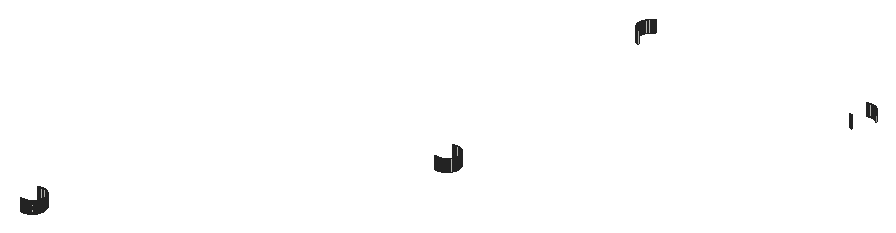
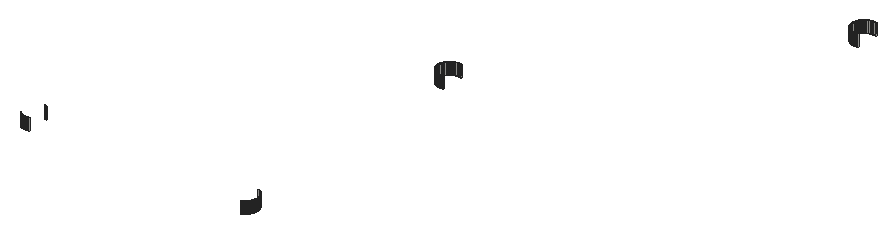
# SketchUp Ruby script. Lengths in inches.
U = 1.inch
M = Sketchup.active_model
def pt(a) = Geom::Point3d.new(a.map { |v| v * U })
def face(e, loops, mat)
  f = e.add_face(loops[0].map { |a| pt(a) })
  loops[1..].each { |l| e.add_face(l.map { |a| pt(a) }).erase! }
  f.material = f.back_material = mat if mat
  f
end
# faces: each face lists its corners as indices into pts; further lists are holes
def faces(e, pts, list, mat = nil) = list.each { |f| face(e, (f[0].is_a?(Array) ? f : [f]).map { |l| l.map { |i| pts[i] } }, mat) }
# xy, xz, yz: faces in a plane at the given z, y or x. An outline is a flat list of corners, or four numbers for a rectangle; further outlines are holes
def ring(l) = l.size == 4 ? [[l[0], l[1]], [l[2], l[1]], [l[2], l[3]], [l[0], l[3]]] : l.each_slice(2).to_a
def flat(e, list, mat, &to3) = list.each { |f| face(e, (f[0].is_a?(Array) ? f : [f]).map { |l| ring(l).map { |u, v| to3.(u, v) } }, mat) }
def xy(e, z, list, mat = nil) = flat(e, list, mat) { |x, y| [x, y, z] }
def xz(e, y, list, mat = nil) = flat(e, list, mat) { |x, z| [x, y, z] }
def yz(e, x, list, mat = nil) = flat(e, list, mat) { |y, z| [x, y, z] }
def lines(e, pts, list) = list.each { |a, b| e.add_line(pt(pts[a]), pt(pts[b])) }
# prism: a flat outline (further loops are holes) pulled along v
def prism(e, loops, v, mat = nil)
  f = face(e, loops, mat); d = Geom::Vector3d.new(v.map { |x| x * U })
  f.pushpull(f.normal.samedirection?(d) ? d.length : -d.length)
end
def box(e, o, s, mat = nil) = prism(e, [[o, [o[0] + s[0], o[1], o[2]], [o[0] + s[0], o[1] + s[1], o[2]], [o[0], o[1] + s[1], o[2]]]], [0, 0, s[2]], mat)
def at(x, y, z, deg = 0) = Geom::Transformation.translation(pt([x, y, z])) * Geom::Transformation.rotation(ORIGIN, Z_AXIS, deg.degrees)
def axes(o, x, y, z) = Geom::Transformation.new([*x, 0, *y, 0, *z, 0, *pt(o).to_a, 1])
def part(name) = M.definitions.add(name)
# library, detail: a bought-in or finely detailed component or shape, given as its bounding box
def library(name, o, s) = part(name).tap { |d| box(d.entities, o, s) }
def detail(e, o, s) = box(e.add_group.entities, o, s)
def put(e, d, t, mat = nil) = e.add_instance(d, t).tap { |i| i.material = mat if mat }
def group(e, t, mat = nil) = e.add_group.tap { |g| g.transformation = t; g.material = mat if mat }.entities
root = M.entities
xz(root,185,[[159.48,231,159.55,234],[159.55,231,159.63,234],[159.63,231,159.71,234]])
xz(root,185.01,[[159.32,231,159.4,234],[159.79,231,159.87,234]])
xz(root,190.99,[[159.33,231,159.41,234],[159.8,231,159.88,234]])
xz(root,191,[[159.49,231,159.57,234],[159.57,231,159.65,234],[159.65,231,159.72,234]])
xz(root,251,[[214.28,231,214.35,234],[214.35,231,214.43,234],[214.43,231,214.51,234]])
xz(root,251.01,[[214.12,231,214.2,234],[214.59,231,214.67,234]])
xz(root,256.99,[[214.13,231,214.21,234],[214.6,231,214.68,234]])
xz(root,257,[[214.29,231,214.37,234],[214.37,231,214.45,234],[214.45,231,214.52,234]])
xz(root,317,[[269.08,231,269.15,234]])
xz(root,317.01,[[268.92,231,269,234]])
xz(root,322.99,[[268.93,231,269.01,234],[269.4,231,269.48,234]])
xz(root,323,[[269.09,231,269.17,234],[269.17,231,269.25,234],[269.25,231,269.32,234]])
yz(root,162.59,[[187.72,231,187.8,234],[188.19,231,188.27,234]])
yz(root,162.6,[[187.875,231,187.95,234],[187.95,231,188.03,234],[188.03,231,188.11,234]])
yz(root,211.4,[[319.89,231,319.97,234],[319.97,231,320.05,234],[320.05,231,320.125,234]])
yz(root,211.41,[[319.73,231,319.81,234],[320.2,231,320.28,234]])
yz(root,217.39,[[253.72,231,253.8,234],[254.19,231,254.27,234]])
yz(root,217.4,[[253.875,231,253.95,234],[253.95,231,254.03,234],[254.03,231,254.11,234]])
p = [[159.09,185.04,231],[159.01,185.06,231],[159.01,185.06,234],[159.09,185.04,234],[159.16,185.03,231],[159.16,185.03,234],
  [159.32,185.01,231],[159.24,185.02,231],[159.24,185.02,234],[159.32,185.01,234],[159.48,185,231],[159.4,185.01,231],
  [159.4,185.01,234],[159.48,185,234],[159.79,185.01,231],[159.71,185,231],[159.71,185,234],[159.79,185.01,234],
  [160.02,185.03,231],[159.95,185.02,231],[159.95,185.02,234],[160.02,185.03,234],[159.87,185.01,231],[159.87,185.01,234],
  [160.1,185.04,231],[160.1,185.04,234],[160.18,185.06,231],[160.18,185.06,234],[158.78,185.11,231],[158.7,185.14,231],
  [158.7,185.14,234],[158.78,185.11,234],[158.86,185.09,231],[158.86,185.09,234],[158.93,185.08,231],[158.93,185.08,234],
  [160.26,185.07,231],[160.26,185.07,234],[160.41,185.11,231],[160.33,185.09,231],[160.33,185.09,234],[160.41,185.11,234],
  [160.48,185.13,231],[160.48,185.13,234],[160.56,185.16,231],[160.56,185.16,234],[160.71,185.21,231],[160.63,185.18,231],
  [160.63,185.18,234],[160.71,185.21,234],[160.78,185.24,231],[160.78,185.24,234],[160.85,185.27,231],[160.85,185.27,234],
  [160.99,185.34,231],[160.92,185.31,231],[160.92,185.31,234],[160.99,185.34,234],[161.0625,185.38,231],[161.0625,185.38,234],
  [161.2,185.46,231],[161.13,185.42,231],[161.13,185.42,234],[161.2,185.46,234],[161.26,185.5,231],[161.26,185.5,234],
  [161.39,185.59,231],[161.33,185.55,231],[161.33,185.55,234],[161.39,185.59,234],[161.45,185.64,231],[161.45,185.64,234],
  [161.51,185.69,231],[161.51,185.69,234],[161.57,185.74,231],[161.57,185.74,234],[161.63,185.79,231],[161.63,185.79,234],
  [161.6875,185.85,231],[161.6875,185.85,234],[161.74,185.9,231],[161.74,185.9,234],[161.8,185.96,231],[161.8,185.96,234],
  [161.85,186.02,231],[161.85,186.02,234],[161.9,186.08,231],[161.9,186.08,234],[161.95,186.14,231],[161.95,186.14,234],
  [162,186.2,231],[162,186.2,234],[162.05,186.26,231],[162.05,186.26,234],[162.09,186.33,231],[162.09,186.33,234],
  [162.13,186.39,231],[162.13,186.39,234],[162.18,186.46,231],[162.18,186.46,234],[162.25,186.6,231],[162.21,186.53,231],
  [162.21,186.53,234],[162.25,186.6,234],[162.29,186.67,231],[162.29,186.67,234],[162.35,186.81,231],[162.32,186.74,231],
  [162.32,186.74,234],[162.35,186.81,234],[162.38,186.88,231],[162.38,186.88,234],[162.41,186.96,231],[162.41,186.96,234],
  [162.46,187.1,231],[162.4375,187.03,231],[162.4375,187.03,234],[162.46,187.1,234],[162.49,187.18,231],[162.49,187.18,234],
  [162.51,187.26,231],[162.51,187.26,234],[162.54,187.41,231],[162.52,187.33,231],[162.52,187.33,234],[162.54,187.41,234],
  [162.56,187.49,231],[162.56,187.49,234],[162.57,187.5625,231],[162.57,187.5625,234],[162.59,187.72,231],[162.58,187.64,231],
  [162.58,187.64,234],[162.59,187.72,234],[162.6,187.875,231],[162.59,187.8,231],[162.59,187.8,234],[162.6,187.875,234],
  [162.59,188.19,231],[162.6,188.11,231],[162.6,188.11,234],[162.59,188.19,234],[162.57,188.42,231],[162.58,188.35,231],
  [162.58,188.35,234],[162.57,188.42,234],[162.59,188.27,231],[162.59,188.27,234],[162.56,188.5,231],[162.56,188.5,234],
  [162.54,188.58,231],[162.54,188.58,234],[162.53,188.66,231],[162.53,188.66,234],[162.49,188.81,231],[162.51,188.73,231],
  [162.51,188.73,234],[162.49,188.81,234],[162.47,188.88,231],[162.47,188.88,234],[162.44,188.96,231],[162.44,188.96,234],
  [162.39,189.11,231],[162.42,189.03,231],[162.42,189.03,234],[162.39,189.11,234],[162.36,189.18,231],[162.36,189.18,234],
  [162.33,189.25,231],[162.33,189.25,234],[162.26,189.39,231],[162.29,189.32,231],[162.29,189.32,234],[162.26,189.39,234],
  [162.22,189.46,231],[162.22,189.46,234],[162.14,189.6,231],[162.18,189.53,231],[162.18,189.53,234],[162.14,189.6,234],
  [162.1,189.66,231],[162.1,189.66,234],[162.01,189.79,231],[162.05,189.73,231],[162.05,189.73,234],[162.01,189.79,234],
  [161.96,189.85,231],[161.96,189.85,234],[161.86,189.97,231],[161.91,189.91,231],[161.91,189.91,234],[161.86,189.97,234],
  [161.75,190.09,231],[161.81,190.03,231],[161.81,190.03,234],[161.75,190.09,234],[161.64,190.2,231],[161.7,190.14,231],
  [161.7,190.14,234],[161.64,190.2,234],[161.58,190.25,231],[161.58,190.25,234],[161.27,190.49,231],[161.34,190.45,231],
  [161.34,190.45,234],[161.27,190.49,234],[161.4,190.4,231],[161.4,190.4,234],[161.14,190.58,231],[161.21,190.53,231],
  [161.21,190.53,234],[161.14,190.58,234],[161,190.65,231],[161.07,190.61,231],[161.07,190.61,234],[161,190.65,234],
  [160.79,190.75,231],[160.86,190.72,231],[160.86,190.72,234],[160.79,190.75,234],[160.93,190.6875,231],[160.93,190.6875,234],
  [160.5,190.86,231],[160.57,190.84,231],[160.57,190.84,234],[160.5,190.86,234],[160.64,190.8125,231],[160.64,190.8125,234],
  [160.72,190.78,231],[160.72,190.78,234],[158.72,190.87,231],[158.79,190.89,231],[158.79,190.89,234],[158.72,190.87,234],
  [158.87,190.91,231],[158.87,190.91,234],[158.94,190.93,231],[158.94,190.93,234],[159.02,190.94,231],[159.02,190.94,234],
  [159.1,190.96,231],[159.1,190.96,234],[160.11,190.96,231],[160.19,190.94,231],[160.19,190.94,234],[160.11,190.96,234],
  [160.27,190.92,231],[160.27,190.92,234],[160.34,190.91,231],[160.34,190.91,234],[160.42,190.89,231],[160.42,190.89,234],
  [159.18,190.97,231],[159.18,190.97,234],[159.25,190.98,231],[159.25,190.98,234],[159.33,190.99,231],[159.33,190.99,234],
  [159.41,190.99,231],[159.49,191,231],[159.49,191,234],[159.41,190.99,234],[159.72,191,231],[159.8,190.99,231],
  [159.8,190.99,234],[159.72,191,234],[159.88,190.99,231],[159.96,190.98,231],[159.96,190.98,234],[159.88,190.99,234],
  [160.04,190.97,231],[160.04,190.97,234],[213.89,251.04,231],[213.81,251.06,231],[213.81,251.06,234],[213.89,251.04,234],
  [213.96,251.03,231],[213.96,251.03,234],[214.12,251.01,231],[214.04,251.02,231],[214.04,251.02,234],[214.12,251.01,234],
  [214.28,251,231],[214.2,251.01,231],[214.2,251.01,234],[214.28,251,234],[214.59,251.01,231],[214.51,251,231],
  [214.51,251,234],[214.59,251.01,234],[214.82,251.03,231],[214.75,251.02,231],[214.75,251.02,234],[214.82,251.03,234],
  [214.67,251.01,231],[214.67,251.01,234],[214.9,251.04,231],[214.9,251.04,234],[214.98,251.06,231],[214.98,251.06,234],
  [213.58,251.11,231],[213.5,251.14,231],[213.5,251.14,234],[213.58,251.11,234],[213.66,251.09,231],[213.66,251.09,234],
  [213.73,251.08,231],[213.73,251.08,234],[215.06,251.07,231],[215.06,251.07,234],[215.21,251.11,231],[215.13,251.09,231],
  [215.13,251.09,234],[215.21,251.11,234],[215.28,251.13,231],[215.28,251.13,234],[215.36,251.16,231],[215.36,251.16,234],
  [215.51,251.21,231],[215.43,251.18,231],[215.43,251.18,234],[215.51,251.21,234],[215.58,251.24,231],[215.58,251.24,234],
  [215.65,251.27,231],[215.65,251.27,234],[215.79,251.34,231],[215.72,251.31,231],[215.72,251.31,234],[215.79,251.34,234],
  [215.86,251.38,231],[215.86,251.38,234],[216,251.46,231],[215.93,251.42,231],[215.93,251.42,234],[216,251.46,234],
  [216.0625,251.5,231],[216.0625,251.5,234],[216.19,251.59,231],[216.125,251.55,231],[216.125,251.55,234],[216.19,251.59,234],
  [216.25,251.64,231],[216.25,251.64,234],[216.3125,251.69,231],[216.3125,251.69,234],[216.375,251.74,231],[216.375,251.74,234],
  [216.43,251.79,231],[216.43,251.79,234],[216.49,251.85,231],[216.49,251.85,234],[216.54,251.9,231],[216.54,251.9,234],
  [216.6,251.96,231],[216.6,251.96,234],[216.65,252.02,231],[216.65,252.02,234],[216.7,252.08,231],[216.7,252.08,234],
  [216.75,252.14,231],[216.75,252.14,234],[216.8,252.2,231],[216.8,252.2,234],[216.85,252.26,231],[216.85,252.26,234],
  [216.89,252.33,231],[216.89,252.33,234],[216.93,252.39,231],[216.93,252.39,234],[216.98,252.46,231],[216.98,252.46,234],
  [217.05,252.6,231],[217.01,252.53,231],[217.01,252.53,234],[217.05,252.6,234],[217.09,252.67,231],[217.09,252.67,234],
  [217.15,252.81,231],[217.12,252.74,231],[217.12,252.74,234],[217.15,252.81,234],[217.18,252.88,231],[217.18,252.88,234],
  [217.21,252.96,231],[217.21,252.96,234],[217.26,253.1,231],[217.24,253.03,231],[217.24,253.03,234],[217.26,253.1,234],
  [217.29,253.18,231],[217.29,253.18,234],[217.31,253.26,231],[217.31,253.26,234],[217.34,253.41,231],[217.32,253.33,231],
  [217.32,253.33,234],[217.34,253.41,234],[217.36,253.49,231],[217.36,253.49,234],[217.37,253.5625,231],[217.37,253.5625,234],
  [217.39,253.72,231],[217.38,253.64,231],[217.38,253.64,234],[217.39,253.72,234],[217.4,253.875,231],[217.39,253.8,231],
  [217.39,253.8,234],[217.4,253.875,234],[217.39,254.19,231],[217.4,254.11,231],[217.4,254.11,234],[217.39,254.19,234],
  [217.37,254.42,231],[217.38,254.35,231],[217.38,254.35,234],[217.37,254.42,234],[217.39,254.27,231],[217.39,254.27,234],
  [217.36,254.5,231],[217.36,254.5,234],[217.34,254.58,231],[217.34,254.58,234],[217.33,254.66,231],[217.33,254.66,234],
  [217.29,254.81,231],[217.31,254.73,231],[217.31,254.73,234],[217.29,254.81,234],[217.27,254.88,231],[217.27,254.88,234],
  [217.24,254.96,231],[217.24,254.96,234],[217.1875,255.11,231],[217.22,255.03,231],[217.22,255.03,234],[217.1875,255.11,234],
  [217.16,255.18,231],[217.16,255.18,234],[217.125,255.25,231],[217.125,255.25,234],[217.06,255.39,231],[217.09,255.32,231],
  [217.09,255.32,234],[217.06,255.39,234],[217.02,255.46,231],[217.02,255.46,234],[216.94,255.6,231],[216.98,255.53,231],
  [216.98,255.53,234],[216.94,255.6,234],[216.9,255.66,231],[216.9,255.66,234],[216.81,255.79,231],[216.85,255.73,231],
  [216.85,255.73,234],[216.81,255.79,234],[216.76,255.85,231],[216.76,255.85,234],[216.66,255.97,231],[216.71,255.91,231],
  [216.71,255.91,234],[216.66,255.97,234],[216.55,256.09,231],[216.61,256.03,231],[216.61,256.03,234],[216.55,256.09,234],
  [216.44,256.2,231],[216.5,256.14,231],[216.5,256.14,234],[216.44,256.2,234],[216.38,256.25,231],[216.38,256.25,234],
  [216.26,256.35,231],[216.32,256.3,231],[216.32,256.3,234],[216.26,256.35,234],[216.07,256.49,231],[216.14,256.45,231],
  [216.14,256.45,234],[216.07,256.49,234],[216.2,256.4,231],[216.2,256.4,234],[215.9375,256.58,231],[216.01,256.53,231],
  [216.01,256.53,234],[215.9375,256.58,234],[215.8,256.65,231],[215.87,256.61,231],[215.87,256.61,234],[215.8,256.65,234],
  [215.59,256.75,231],[215.66,256.72,231],[215.66,256.72,234],[215.59,256.75,234],[215.73,256.6875,231],[215.73,256.6875,234],
  [215.3,256.86,231],[215.37,256.84,231],[215.37,256.84,234],[215.3,256.86,234],[215.44,256.8125,231],[215.44,256.8125,234],
  [215.52,256.78,231],[215.52,256.78,234],[213.52,256.87,231],[213.59,256.89,231],[213.59,256.89,234],[213.52,256.87,234],
  [213.67,256.91,231],[213.67,256.91,234],[213.74,256.93,231],[213.74,256.93,234],[213.82,256.94,231],[213.82,256.94,234],
  [213.9,256.96,231],[213.9,256.96,234],[214.91,256.96,231],[214.99,256.94,231],[214.99,256.94,234],[214.91,256.96,234],
  [215.07,256.92,231],[215.07,256.92,234],[215.14,256.91,231],[215.14,256.91,234],[215.22,256.89,231],[215.22,256.89,234],
  [213.98,256.97,231],[213.98,256.97,234],[214.05,256.98,231],[214.05,256.98,234],[214.13,256.99,231],[214.13,256.99,234],
  [214.21,256.99,231],[214.29,257,231],[214.29,257,234],[214.21,256.99,234],[214.52,257,231],[214.6,256.99,231],
  [214.6,256.99,234],[214.52,257,234],[214.68,256.99,231],[214.76,256.98,231],[214.76,256.98,234],[214.68,256.99,234],
  [214.84,256.97,231],[214.84,256.97,234],[268.6875,317.04,231],[268.61,317.06,231],[268.61,317.06,234],[268.6875,317.04,234],
  [268.76,317.03,231],[268.76,317.03,234],[268.92,317.01,231],[268.84,317.02,231],[268.84,317.02,234],[268.92,317.01,234],
  [269.08,317,231],[269,317.01,231],[269,317.01,234],[269.08,317,234],[213.5,317.14,231],[213.43,317.16,231],
  [213.43,317.16,234],[213.5,317.14,234],[268.38,317.11,231],[268.3,317.14,231],[268.3,317.14,234],[268.38,317.11,234],
  [268.46,317.09,231],[268.46,317.09,234],[268.53,317.08,231],[268.53,317.08,234],[213.21,317.25,231],[213.14,317.28,231],
  [213.14,317.28,234],[213.21,317.25,234],[213.28,317.22,231],[213.28,317.22,234],[213.36,317.1875,231],[213.36,317.1875,234],
  [213,317.35,231],[212.93,317.39,231],[212.93,317.39,234],[213,317.35,234],[213.07,317.3125,231],[213.07,317.3125,234],
  [212.86,317.42,231],[212.79,317.47,231],[212.79,317.47,234],[212.86,317.42,234],[212.73,317.51,231],[212.73,317.51,234],
  [212.66,317.55,231],[212.66,317.55,234],[212.6,317.6,231],[212.54,317.65,231],[212.54,317.65,234],[212.6,317.6,234],
  [212.48,317.7,231],[212.48,317.7,234],[212.42,317.75,231],[212.42,317.75,234],[212.36,317.8,231],[212.36,317.8,234],
  [212.3,317.86,231],[212.3,317.86,234],[212.25,317.91,231],[212.25,317.91,234],[212.19,317.97,231],[212.19,317.97,234],
  [212.14,318.03,231],[212.14,318.03,234],[212.09,318.09,231],[212.09,318.09,234],[212.04,318.15,231],[212.04,318.15,234],
  [211.99,318.21,231],[211.99,318.21,234],[211.95,318.27,231],[211.95,318.27,234],[211.9,318.34,231],[211.9,318.34,234],
  [211.86,318.4,231],[211.86,318.4,234],[211.82,318.47,231],[211.82,318.47,234],[211.78,318.54,231],[211.74,318.61,231],
  [211.74,318.61,234],[211.78,318.54,234],[211.71,318.68,231],[211.71,318.68,234],[211.67,318.75,231],[211.64,318.82,231],
  [211.64,318.82,234],[211.67,318.75,234],[211.61,318.89,231],[211.61,318.89,234],[211.58,318.97,231],[211.58,318.97,234],
  [211.56,319.04,231],[211.53,319.12,231],[211.53,319.12,234],[211.56,319.04,234],[211.51,319.19,231],[211.51,319.19,234],
  [211.49,319.27,231],[211.49,319.27,234],[211.47,319.34,231],[211.47,319.34,234],[211.46,319.42,231],[211.46,319.42,234],
  [211.44,319.5,231],[211.44,319.5,234],[211.43,319.58,231],[211.43,319.58,234],[211.42,319.65,231],[211.42,319.65,234],
  [211.41,319.73,231],[211.41,319.73,234],[211.41,319.81,231],[211.4,319.89,231],[211.4,319.89,234],[211.41,319.81,234],
  [211.4,320.125,231],[211.41,320.2,231],[211.41,320.2,234],[211.4,320.125,234],[211.41,320.28,231],[211.42,320.36,231],
  [211.42,320.36,234],[211.41,320.28,234],[211.43,320.4375,231],[211.43,320.4375,234],[211.44,320.51,231],[211.44,320.51,234],
  [211.46,320.59,231],[211.46,320.59,234],[211.48,320.67,231],[211.48,320.67,234],[211.49,320.74,231],[211.49,320.74,234],
  [211.51,320.82,231],[211.51,320.82,234],[211.54,320.9,231],[211.54,320.9,234],[211.5625,320.97,231],[211.5625,320.97,234],
  [211.59,321.04,231],[211.59,321.04,234],[211.62,321.12,231],[211.62,321.12,234],[211.65,321.19,231],[211.65,321.19,234],
  [211.68,321.26,231],[211.68,321.26,234],[211.71,321.33,231],[211.71,321.33,234],[211.75,321.4,231],[211.75,321.4,234],
  [211.79,321.47,231],[211.79,321.47,234],[211.82,321.54,231],[211.82,321.54,234],[211.87,321.61,231],[211.87,321.61,234],
  [211.91,321.67,231],[211.91,321.67,234],[211.95,321.74,231],[211.95,321.74,234],[212,321.8,231],[212,321.8,234],
  [212.05,321.86,231],[212.05,321.86,234],[212.1,321.92,231],[212.1,321.92,234],[212.15,321.98,231],[212.15,321.98,234],
  [212.2,322.04,231],[212.2,322.04,234],[212.26,322.1,231],[212.26,322.1,234],[212.3125,322.15,231],[212.3125,322.15,234],
  [212.37,322.21,231],[212.37,322.21,234],[212.43,322.26,231],[212.43,322.26,234],[212.49,322.31,231],[212.49,322.31,234],
  [212.55,322.36,231],[212.55,322.36,234],[271.0625,322.35,231],[271.12,322.3,231],[271.12,322.3,234],[271.0625,322.35,234],
  [271.18,322.25,231],[271.18,322.25,234],[212.61,322.41,231],[212.61,322.41,234],[212.67,322.45,231],[212.67,322.45,234],
  [270.87,322.49,231],[270.9375,322.45,231],[270.9375,322.45,234],[270.87,322.49,234],[271,322.4,231],[271,322.4,234],
  [212.74,322.5,231],[212.74,322.5,234],[212.8,322.54,231],[212.8,322.54,234],[212.87,322.58,231],[212.87,322.58,234],
  [270.74,322.58,231],[270.81,322.53,231],[270.81,322.53,234],[270.74,322.58,234],[212.9375,322.62,231],[212.9375,322.62,234],
  [213.01,322.66,231],[213.01,322.66,234],[270.6,322.65,231],[270.67,322.61,231],[270.67,322.61,234],[270.6,322.65,234],
  [213.08,322.69,231],[213.08,322.69,234],[213.15,322.73,231],[213.15,322.73,234],[213.22,322.76,231],[213.22,322.76,234],
  [270.39,322.75,231],[270.46,322.72,231],[270.46,322.72,234],[270.39,322.75,234],[270.53,322.6875,231],[270.53,322.6875,234],
  [213.29,322.79,231],[213.29,322.79,234],[213.37,322.82,231],[213.37,322.82,234],[213.44,322.84,231],[213.44,322.84,234],
  [213.52,322.87,231],[213.52,322.87,234],[270.1,322.86,231],[270.17,322.84,231],[270.17,322.84,234],[270.1,322.86,234],
  [270.24,322.8125,231],[270.24,322.8125,234],[270.32,322.78,231],[270.32,322.78,234],[268.32,322.87,231],[268.39,322.89,231],
  [268.39,322.89,234],[268.32,322.87,234],[268.47,322.91,231],[268.47,322.91,234],[268.54,322.93,231],[268.54,322.93,234],
  [268.62,322.94,231],[268.62,322.94,234],[268.7,322.96,231],[268.7,322.96,234],[269.71,322.96,231],[269.79,322.94,231],
  [269.79,322.94,234],[269.71,322.96,234],[269.87,322.92,231],[269.87,322.92,234],[269.94,322.91,231],[269.94,322.91,234],
  [270.02,322.89,231],[270.02,322.89,234],[268.78,322.97,231],[268.78,322.97,234],[268.85,322.98,231],[268.85,322.98,234],
  [268.93,322.99,231],[268.93,322.99,234],[269.01,322.99,231],[269.09,323,231],[269.09,323,234],[269.01,322.99,234],
  [269.32,323,231],[269.4,322.99,231],[269.4,322.99,234],[269.32,323,234],[269.48,322.99,231],[269.56,322.98,231],
  [269.56,322.98,234],[269.48,322.99,234],[269.64,322.97,231],[269.64,322.97,234]]
faces(root,p,[[0,1,2,3],[4,0,3,5],[6,7,8,9],[7,4,5,8],[10,11,12,13],[14,15,16,17],[18,19,20,21],[19,22,23,20],
  [24,18,21,25],[26,24,25,27],[28,29,30,31],[32,28,31,33],[1,34,35,2],[34,32,33,35],[36,26,27,37],[38,39,40,41],
  [39,36,37,40],[42,38,41,43],[44,42,43,45],[46,47,48,49],[47,44,45,48],[50,46,49,51],[52,50,51,53],[54,55,56,57],
  [55,52,53,56],[58,54,57,59],[60,61,62,63],[61,58,59,62],[64,60,63,65],[66,67,68,69],[67,64,65,68],[70,66,69,71],
  [72,70,71,73],[74,72,73,75],[76,74,75,77],[78,76,77,79],[80,78,79,81],[82,80,81,83],[84,82,83,85],[86,84,85,87],
  [88,86,87,89],[90,88,89,91],[92,90,91,93],[94,92,93,95],[96,94,95,97],[98,96,97,99],[100,101,102,103],[101,98,99,102],
  [104,100,103,105],[106,107,108,109],[107,104,105,108],[110,106,109,111],[112,110,111,113],[114,115,116,117],[115,112,113,116],[118,114,117,119],
  [120,118,119,121],[122,123,124,125],[123,120,121,124],[126,122,125,127],[128,126,127,129],[130,131,132,133],[131,128,129,132],[134,135,136,137],
  [138,139,140,141],[142,143,144,145],[143,146,147,144],[148,142,145,149],[150,148,149,151],[152,150,151,153],[154,155,156,157],[155,152,153,156],
  [158,154,157,159],[160,158,159,161],[162,163,164,165],[163,160,161,164],[166,162,165,167],[168,166,167,169],[170,171,172,173],[171,168,169,172],
  [174,170,173,175],[176,177,178,179],[177,174,175,178],[180,176,179,181],[182,183,184,185],[183,180,181,184],[186,182,185,187],[188,189,190,191],
  [189,186,187,190],[192,193,194,195],[193,188,191,194],[196,197,198,199],[197,192,195,198],[200,196,199,201],[202,203,204,205],[203,206,207,204],
  [208,209,210,211],[209,202,205,210],[212,213,214,215],[213,208,211,214],[216,217,218,219],[217,220,221,218],[220,212,215,221],[222,223,224,225],
  [223,226,227,224],[226,228,229,227],[228,216,219,229],[230,231,232,233],[231,234,235,232],[234,236,237,235],[236,238,239,237],[238,240,241,239],
  [242,243,244,245],[243,246,247,244],[246,248,249,247],[248,250,251,249],[250,222,225,251],[240,252,253,241],[252,254,255,253],[254,256,257,255],
  [258,259,260,261],[262,263,264,265],[266,267,268,269],[267,270,271,268],[270,242,245,271],[272,273,274,275],[276,272,275,277],[278,279,280,281],
  [279,276,277,280],[282,283,284,285],[286,287,288,289],[290,291,292,293],[291,294,295,292],[296,290,293,297],[298,296,297,299],[300,301,302,303],
  [304,300,303,305],[273,306,307,274],[306,304,305,307],[308,298,299,309],[310,311,312,313],[311,308,309,312],[314,310,313,315],[316,314,315,317],
  [318,319,320,321],[319,316,317,320],[322,318,321,323],[324,322,323,325],[326,327,328,329],[327,324,325,328],[330,326,329,331],[332,333,334,335],
  [333,330,331,334],[336,332,335,337],[338,339,340,341],[339,336,337,340],[342,338,341,343],[344,342,343,345],[346,344,345,347],[348,346,347,349],
  [350,348,349,351],[352,350,351,353],[354,352,353,355],[356,354,355,357],[358,356,357,359],[360,358,359,361],[362,360,361,363],[364,362,363,365],
  [366,364,365,367],[368,366,367,369],[370,368,369,371],[372,373,374,375],[373,370,371,374],[376,372,375,377],[378,379,380,381],[379,376,377,380],
  [382,378,381,383],[384,382,383,385],[386,387,388,389],[387,384,385,388],[390,386,389,391],[392,390,391,393],[394,395,396,397],[395,392,393,396],
  [398,394,397,399],[400,398,399,401],[402,403,404,405],[403,400,401,404],[406,407,408,409],[410,411,412,413],[414,415,416,417],[415,418,419,416],
  [420,414,417,421],[422,420,421,423],[424,422,423,425],[426,427,428,429],[427,424,425,428],[430,426,429,431],[432,430,431,433],[434,435,436,437],
  [435,432,433,436],[438,434,437,439],[440,438,439,441],[442,443,444,445],[443,440,441,444],[446,442,445,447],[448,449,450,451],[449,446,447,450],
  [452,448,451,453],[454,455,456,457],[455,452,453,456],[458,454,457,459],[460,461,462,463],[461,458,459,462],[464,465,466,467],[465,460,463,466],
  [468,469,470,471],[469,464,467,470],[472,468,471,473],[474,475,476,477],[475,472,473,476],[478,479,480,481],[479,482,483,480],[482,474,477,483],
  [484,485,486,487],[485,478,481,486],[488,489,490,491],[489,484,487,490],[492,493,494,495],[493,496,497,494],[496,488,491,497],[498,499,500,501],
  [499,502,503,500],[502,504,505,503],[504,492,495,505],[506,507,508,509],[507,510,511,508],[510,512,513,511],[512,514,515,513],[514,516,517,515],
  [518,519,520,521],[519,522,523,520],[522,524,525,523],[524,526,527,525],[526,498,501,527],[516,528,529,517],[528,530,531,529],[530,532,533,531],
  [534,535,536,537],[538,539,540,541],[542,543,544,545],[543,546,547,544],[546,518,521,547],[548,549,550,551],[552,548,551,553],[554,555,556,557],
  [555,552,553,556],[558,559,560,561],[562,563,564,565],[566,567,568,569],[570,566,569,571],[549,572,573,550],[572,570,571,573],[574,575,576,577],
  [578,574,577,579],[580,578,579,581],[563,580,581,564],[582,583,584,585],[586,582,585,587],[575,586,587,576],[588,589,590,591],[583,588,591,584],
  [589,592,593,590],[592,594,595,593],[596,597,598,599],[597,600,601,598],[594,596,599,595],[600,602,603,601],[602,604,605,603],[604,606,607,605],
  [606,608,609,607],[608,610,611,609],[610,612,613,611],[612,614,615,613],[614,616,617,615],[616,618,619,617],[618,620,621,619],[620,622,623,621],
  [622,624,625,623],[624,626,627,625],[628,629,630,631],[626,628,631,627],[629,632,633,630],[634,635,636,637],[632,634,637,633],[635,638,639,636],
  [638,640,641,639],[642,643,644,645],[640,642,645,641],[643,646,647,644],[646,648,649,647],[648,650,651,649],[650,652,653,651],[652,654,655,653],
  [654,656,657,655],[656,658,659,657],[658,660,661,659],[662,663,664,665],[666,667,668,669],[670,671,672,673],[671,674,675,672],[674,676,677,675],
  [676,678,679,677],[678,680,681,679],[680,682,683,681],[682,684,685,683],[684,686,687,685],[686,688,689,687],[688,690,691,689],[690,692,693,691],
  [692,694,695,693],[694,696,697,695],[696,698,699,697],[698,700,701,699],[700,702,703,701],[702,704,705,703],[704,706,707,705],[706,708,709,707],
  [708,710,711,709],[710,712,713,711],[712,714,715,713],[714,716,717,715],[716,718,719,717],[718,720,721,719],[720,722,723,721],[722,724,725,723],
  [724,726,727,725],[726,728,729,727],[728,730,731,729],[730,732,733,731],[734,735,736,737],[735,738,739,736],[732,740,741,733],[740,742,743,741],
  [744,745,746,747],[745,748,749,746],[748,734,737,749],[742,750,751,743],[750,752,753,751],[752,754,755,753],[756,757,758,759],[757,744,747,758],
  [754,760,761,755],[760,762,763,761],[764,765,766,767],[765,756,759,766],[762,768,769,763],[768,770,771,769],[770,772,773,771],[774,775,776,777],
  [775,778,779,776],[778,764,767,779],[772,780,781,773],[780,782,783,781],[782,784,785,783],[784,786,787,785],[788,789,790,791],[789,792,793,790],
  [792,794,795,793],[794,774,777,795],[796,797,798,799],[797,800,801,798],[800,802,803,801],[802,804,805,803],[804,806,807,805],[808,809,810,811],
  [809,812,813,810],[812,814,815,813],[814,816,817,815],[816,788,791,817],[806,818,819,807],[818,820,821,819],[820,822,823,821],[824,825,826,827],
  [828,829,830,831],[832,833,834,835],[833,836,837,834],[836,808,811,837]])
